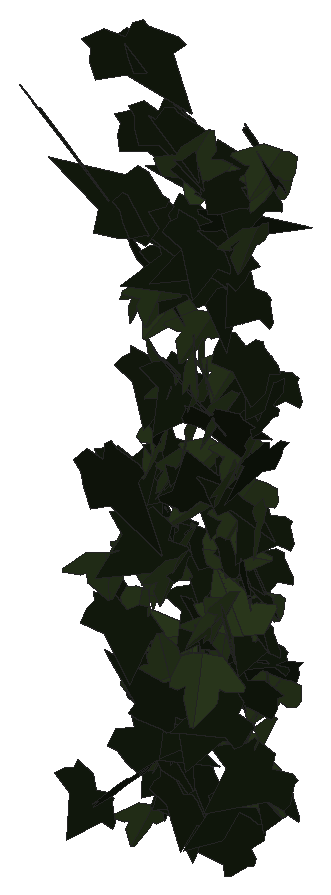
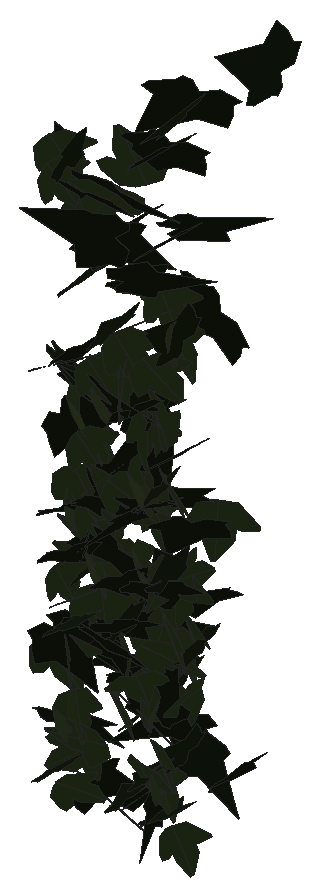
# SketchUp Ruby script. Lengths in inches.
U = 1.inch
M = Sketchup.active_model
def pt(a) = Geom::Point3d.new(a.map { |v| v * U })
def face(e, loops, mat)
  f = e.add_face(loops[0].map { |a| pt(a) })
  loops[1..].each { |l| e.add_face(l.map { |a| pt(a) }).erase! }
  f.material = f.back_material = mat if mat
  f
end
# faces: each face lists its corners as indices into pts; further lists are holes
def faces(e, pts, list, mat = nil) = list.each { |f| face(e, (f[0].is_a?(Array) ? f : [f]).map { |l| l.map { |i| pts[i] } }, mat) }
# xy, xz, yz: faces in a plane at the given z, y or x. An outline is a flat list of corners, or four numbers for a rectangle; further outlines are holes
def ring(l) = l.size == 4 ? [[l[0], l[1]], [l[2], l[1]], [l[2], l[3]], [l[0], l[3]]] : l.each_slice(2).to_a
def flat(e, list, mat, &to3) = list.each { |f| face(e, (f[0].is_a?(Array) ? f : [f]).map { |l| ring(l).map { |u, v| to3.(u, v) } }, mat) }
def xy(e, z, list, mat = nil) = flat(e, list, mat) { |x, y| [x, y, z] }
def xz(e, y, list, mat = nil) = flat(e, list, mat) { |x, z| [x, y, z] }
def yz(e, x, list, mat = nil) = flat(e, list, mat) { |y, z| [x, y, z] }
def lines(e, pts, list) = list.each { |a, b| e.add_line(pt(pts[a]), pt(pts[b])) }
# prism: a flat outline (further loops are holes) pulled along v
def prism(e, loops, v, mat = nil)
  f = face(e, loops, mat); d = Geom::Vector3d.new(v.map { |x| x * U })
  f.pushpull(f.normal.samedirection?(d) ? d.length : -d.length)
end
def box(e, o, s, mat = nil) = prism(e, [[o, [o[0] + s[0], o[1], o[2]], [o[0] + s[0], o[1] + s[1], o[2]], [o[0], o[1] + s[1], o[2]]]], [0, 0, s[2]], mat)
def at(x, y, z, deg = 0) = Geom::Transformation.translation(pt([x, y, z])) * Geom::Transformation.rotation(ORIGIN, Z_AXIS, deg.degrees)
def axes(o, x, y, z) = Geom::Transformation.new([*x, 0, *y, 0, *z, 0, *pt(o).to_a, 1])
def part(name) = M.definitions.add(name)
# library, detail: a bought-in or finely detailed component or shape, given as its bounding box
def library(name, o, s) = part(name).tap { |d| box(d.entities, o, s) }
def detail(e, o, s) = box(e.add_group.entities, o, s)
def put(e, d, t, mat = nil) = e.add_instance(d, t).tap { |i| i.material = mat if mat }
def group(e, t, mat = nil) = e.add_group.tap { |g| g.transformation = t; g.material = mat if mat }.entities
root = M.entities
M.materials.add("1026 AP 7946 SUNNY SIDE UP").color = [254, 231, 186]
M.materials.add("efeu1").color = [18, 25, 13]
M.materials.add("efeu2").color = [43, 57, 29]
c1 = part("ivyleaf_9")
p = [[1.54,2.16,1.25],[1.36,2.04,1.19],[-0.21,0.99,0.68],[-0.71,1.11,0.82],[-0.85,0.86,0.67],[-0.8,0.17,0.21],
  [-0.9,-0.01,0.1],[-0.67,-0.16,-0.02],[-0.08,-0.08,-0.05],[-0.03,-0.6,-0.4],[0.65,-0.88,-0.66],[0.83,-0.6,-0.49],
  [1.29,-0.42,-0.43],[1.8125,-0.07,-0.26],[1.21,0.44,0.15]]
faces(c1.entities,p,[[0,1,2,3,4,5,6,7,8,9,10,11,12,13,14]],"efeu1")
c2 = part("ivyleaf_10")
p = [[0,0.5,-0.03],[-0.0625,2.02,-0.43],[-0.19,2.01,-0.46],[-0.54,1.05,-0.29],[-0.52,0.625,-0.18],[-0.83,0.76,-0.28],
  [-1.16,0.64,-0.33],[-1.15,0.33,-0.24],[-0.77,-0.39,0.02],[-0.3,-0.51,0.16],[0.04,-0.48,0.23],[-0.02,2.01,-0.4375],
  [-0.06,2.01,-0.43],[0.04,-0.49,0.23],[0.67,-0.49,0.14],[1.38,0.36,-0.2],[1.375,0.51,-0.24],[0.81,0.65,-0.19],
  [0.62,0.59,-0.15],[0.6,1.09,-0.28],[0.5,1.23,-0.31]]
faces(c2.entities,p,[[0,1,2,3,4,5,6,7,8,9,10],[11,12,0,13,14,15,16,17,18,19,20]],"efeu2")
put(root,c1,axes([110.82,211.98,271.07],[0.22483,-0.24463,-0.03492],[-0.03089,0.02617,-0.29173],[0.3868,0.14428,-0.003]),"1026 AP 7946 SUNNY SIDE UP")
put(root,c1,axes([110.93,212.53,274.21],[-0.10088,-0.26489,0.10822],[-0.00053,-0.10914,-0.28036],[0.44895,-0.05965,0.02399]),"1026 AP 7946 SUNNY SIDE UP")
put(root,c1,axes([110.88,212.15,273.02],[-0.12749,-0.24464,-0.16443],[0.11207,0.14259,-0.26392],[0.44419,-0.10619,0.01939]),"1026 AP 7946 SUNNY SIDE UP")
put(root,c2,axes([111.05,212.09,272.0625],[0.02647,-0.03472,0.31078],[0.08986,-0.29657,-0.04015],[0.46926,0.05875,-0.00984]),"1026 AP 7946 SUNNY SIDE UP")
put(root,c1,axes([111.05,211.11,268.53],[-0.12847,-0.24075,0.1698],[-0.07523,-0.15923,-0.26279],[0.45379,-0.09456,0.00451]),"1026 AP 7946 SUNNY SIDE UP")
put(root,c1,axes([110.87,212.26,269.49],[0.16139,-0.23387,0.08171],[0.03475,-0.07829,-0.26334],[0.38743,0.10445,-0.01042]),"1026 AP 7946 SUNNY SIDE UP")
put(root,c2,axes([111.14,212.125,275.85],[0.01915,-0.31792,0.0495],[0.00358,-0.0498,-0.32805],[0.50599,0.01238,0.00045]),"1026 AP 7946 SUNNY SIDE UP")
put(root,c1,axes([111.45,211.65,277.25],[-0.30448,-0.25939,-0.13736],[-0.14977,-0.09316,0.33235],[-0.43234,0.21496,-0.01839]),"1026 AP 7946 SUNNY SIDE UP")
put(root,c2,axes([111.19,212.23,271.29],[0.24303,-0.2311,-0.07092],[-0.06134,0.05515,-0.28608],[0.37357,0.1594,-0.00084]),"1026 AP 7946 SUNNY SIDE UP")
put(root,c2,axes([111.08,211.8,270.11],[0.03825,-0.06161,-0.3049],[0.13909,0.28502,-0.05203],[0.45399,-0.08213,0.04163]),"1026 AP 7946 SUNNY SIDE UP")
put(root,c1,axes([110.875,212.39,276.02],[0.21679,-0.26213,0.13752],[0.08115,-0.12525,-0.30562],[0.45645,0.14677,-0.01098]),"1026 AP 7946 SUNNY SIDE UP")
put(root,c1,axes([110.97,212.55,272.3125],[0.02608,-0.19739,0.20165],[0.09253,-0.19029,-0.20278],[0.42847,0.05311,0.03151]),"1026 AP 7946 SUNNY SIDE UP")
put(root,c2,axes([111.25,212,267.9],[-0.15086,-0.24891,0.06861],[-0.02033,-0.06784,-0.27493],[0.40522,-0.09607,0.01175]),"1026 AP 7946 SUNNY SIDE UP")
put(root,c2,axes([111.3125,212.49,275.45],[-0.23769,-0.19774,0.18427],[-0.0587,-0.18912,-0.24746],[0.41633,-0.13956,0.07031]),"1026 AP 7946 SUNNY SIDE UP")
put(root,c1,axes([111.01,212.15,279.43],[0.23464,-0.27386,-0.07967],[-0.04055,0.07219,-0.32065],[0.44496,0.15099,0.0128]),"1026 AP 7946 SUNNY SIDE UP")
put(root,c1,axes([111.23,212.42,268.38],[-0.18187,-0.17107,0.16776],[0.00156,-0.18265,-0.19685],[0.37243,-0.08278,0.08275]),"1026 AP 7946 SUNNY SIDE UP")
put(root,c2,axes([111.39,211.96,271.86],[-0.50214,-0.04065,0.04773],[-0.06554,-0.03932,-0.33009],[0.07177,-0.32032,0.03253]),"1026 AP 7946 SUNNY SIDE UP")
put(root,c2,axes([111.33,212.25,268.89],[-0.00042,-0.29262,0.02638],[-0.00053,-0.02727,-0.30162],[0.46212,-0.0003,-0.00032]),"1026 AP 7946 SUNNY SIDE UP")
put(root,c1,axes([111.05,211.83,279.6],[-0.08354,-0.17438,-0.31942],[0.18521,0.28613,-0.18549],[0.52636,-0.12836,0.01457]),"1026 AP 7946 SUNNY SIDE UP")
put(root,c1,axes([111.27,212.48,272.05],[-0.2802,-0.22211,-0.04672],[0.06855,0.02141,-0.29248],[0.34941,-0.18232,0.01991]),"1026 AP 7946 SUNNY SIDE UP")
put(root,c2,axes([111.24,212.22,273.58],[0.32756,-0.2155,0.10995],[0.07975,-0.10029,-0.30768],[0.3705,0.21211,-0.03098]),"1026 AP 7946 SUNNY SIDE UP")
put(root,c2,axes([111.375,211.74,270.77],[0.10766,-0.28193,0.00565],[-0.00779,-0.0085,-0.29885],[0.44337,0.06831,-0.00662]),"1026 AP 7946 SUNNY SIDE UP")
put(root,c2,axes([111.4,212.24,269.3125],[0.2735,-0.1933,-0.0689],[-0.07163,0.0475,-0.26761],[0.31298,0.17979,-0.00103]),"1026 AP 7946 SUNNY SIDE UP")
put(root,c2,axes([111.35,212.06,272.08],[-0.10457,-0.21622,-0.22476],[0.10442,0.20654,-0.23183],[0.47016,-0.09396,0.0015]),"1026 AP 7946 SUNNY SIDE UP")
put(root,c2,axes([111.64,212.04,270.67],[-0.20058,0.01867,0.24939],[-0.29674,-0.17951,-0.08927],[0.23994,-0.20639,0.09807]),"1026 AP 7946 SUNNY SIDE UP")
put(root,c2,axes([111.27,211.74,271.24],[0.34499,-0.16401,0.14469],[0.14626,-0.11037,-0.28125],[0.30747,0.23652,-0.02856]),"1026 AP 7946 SUNNY SIDE UP")
put(root,c1,axes([111.59,211.15,268.87],[-0.16544,0.29418,-0.12402],[0.04198,-0.11994,-0.32224],[-0.49905,-0.10762,0.01401]),"1026 AP 7946 SUNNY SIDE UP")
put(root,c2,axes([111.1875,212.32,274.375],[-0.25193,0.10093,0.2724],[0.36559,-0.12516,0.19405],[0.25227,0.28217,-0.00918]),"1026 AP 7946 SUNNY SIDE UP")
put(root,c1,axes([111.02,210.1,279.2],[0.33578,-0.29164,0.19388],[0.1489,-0.16564,-0.37283],[0.52653,0.23283,-0.0182]),"1026 AP 7946 SUNNY SIDE UP")
put(root,c1,axes([111.53,212.12,268.46],[0.06782,-0.06736,-0.30721],[-0.34267,0.20388,-0.07883],[0.33629,0.22133,-0.01837]),"1026 AP 7946 SUNNY SIDE UP")
put(root,c1,axes([111.41,212.12,273.68],[0.03377,0.209,0.21516],[-0.14806,-0.19243,0.20841],[0.43898,-0.08098,0.05375]),"1026 AP 7946 SUNNY SIDE UP")
put(root,c2,axes([111.42,212.3,270.09],[-0.19323,0.22713,-0.09072],[0.04701,-0.08527,-0.26618],[-0.38089,-0.12575,0.01317]),"1026 AP 7946 SUNNY SIDE UP")
put(root,c1,axes([111.82,212.38,276.6],[-0.23655,0.01336,0.28194],[-0.41882,-0.08,-0.14732],[0.10055,-0.30181,0.04963]),"1026 AP 7946 SUNNY SIDE UP")
put(root,c1,axes([111.35,212.4375,273.39],[-0.0308,-0.22698,0.20443],[0.008,-0.20037,-0.23524],[0.47534,-0.01134,0.01721]),"1026 AP 7946 SUNNY SIDE UP")
put(root,c1,axes([111.29,211.77,270.31],[0.20454,-0.25715,-0.01721],[-0.02181,0.01006,-0.29671],[0.40446,0.13059,-0.0073]),"1026 AP 7946 SUNNY SIDE UP")
put(root,c2,axes([111.53,210.76,272.35],[-0.3134,-0.25493,-0.03631],[0.05081,0.01759,-0.33293],[0.40116,-0.20139,0.0138]),"1026 AP 7946 SUNNY SIDE UP")
put(root,c1,axes([111.54,212.125,269.84],[0.33563,-0.12698,0.14382],[-0.16714,0.09455,0.25527],[-0.24619,-0.2373,0.02275]),"1026 AP 7946 SUNNY SIDE UP")
put(root,c2,axes([111.55,212.26,274.41],[-0.16161,-0.27546,-0.04722],[0.0479,0.03582,-0.30224],[0.43607,-0.10602,0.01569]),"1026 AP 7946 SUNNY SIDE UP")
put(root,c2,axes([111.5,212.38,269.02],[0.38132,-0.11167,0.00637],[-0.00344,-0.02101,-0.27439],[0.17588,0.24169,-0.01919]),"1026 AP 7946 SUNNY SIDE UP")
put(root,c1,axes([111.45,211.29,271.29],[-0.14008,-0.29047,-0.03741],[0.04419,0.02757,-0.31224],[0.45784,-0.09153,0.01869]),"1026 AP 7946 SUNNY SIDE UP")
put(root,c1,axes([111.33,211.72,277.28],[0.19142,-0.2494,-0.13753],[0.00345,0.14468,-0.2785],[0.44375,0.10646,0.0615]),"1026 AP 7946 SUNNY SIDE UP")
put(root,c1,axes([111.38,212.36,269.02],[0.07782,-0.25434,0.06433],[0.0399,-0.06006,-0.26694],[0.41041,0.05406,0.01375]),"1026 AP 7946 SUNNY SIDE UP")
put(root,c1,axes([111.54,212.38,276.07],[-0.17902,-0.2306,0.14655],[-0.00973,-0.15343,-0.25983],[0.42702,-0.10017,0.05552]),"1026 AP 7946 SUNNY SIDE UP")
put(root,c1,axes([111.63,212.4,273.08],[-0.25672,-0.19054,0.14646],[-0.05548,-0.15239,-0.25115],[0.3707,-0.15476,0.06384]),"1026 AP 7946 SUNNY SIDE UP")
put(root,c2,axes([111.6875,211.74,276.12],[-0.18772,-0.27489,0.07302],[-0.01104,-0.0757,-0.30828],[0.44686,-0.11735,0.02306]),"1026 AP 7946 SUNNY SIDE UP")
put(root,c2,axes([111.66,212.12,273.32],[0.03751,-0.24578,0.1633],[0.0337,-0.15855,-0.25527],[0.45983,0.03167,0.00539]),"1026 AP 7946 SUNNY SIDE UP")
put(root,c2,axes([111.63,212.38,270.4],[0.28623,0.18692,-0.08485],[-0.05919,-0.07916,-0.26781],[-0.31636,0.18392,-0.02666]),"1026 AP 7946 SUNNY SIDE UP")
put(root,c2,axes([111.6,212.5,273.63],[0.14543,-0.19341,0.21253],[0.15147,-0.18376,-0.22186],[0.4194,0.13343,0.00643]),"1026 AP 7946 SUNNY SIDE UP")
put(root,c2,axes([111.64,212.14,269.93],[0.02505,-0.20313,0.22256],[0.12174,-0.20717,-0.20666],[0.45147,0.06713,0.04338]),"1026 AP 7946 SUNNY SIDE UP")
put(root,c2,axes([111.91,211.74,270.04],[-0.23993,-0.10944,0.2045],[-0.21514,-0.14725,-0.19224],[0.28526,-0.20311,0.02702]),"1026 AP 7946 SUNNY SIDE UP")
put(root,c1,axes([111.53,211.91,278.6],[0.12207,-0.29747,-0.09822],[0.02937,0.10077,-0.31321],[0.48949,0.06814,0.04329]),"1026 AP 7946 SUNNY SIDE UP")
put(root,c1,axes([111.51,211.46,269.48],[0.15298,-0.07527,-0.30834],[0.04638,0.31425,-0.0698],[0.48241,-0.00634,0.10449]),"1026 AP 7946 SUNNY SIDE UP")
put(root,c1,axes([111.75,212.22,268.43],[-0.16228,-0.1635,0.22591],[-0.08531,-0.21847,-0.19458],[0.42275,-0.10685,0.04746]),"1026 AP 7946 SUNNY SIDE UP")
put(root,c2,axes([111.77,212.18,272.17],[0.13474,-0.27024,0.06167],[0.02193,-0.05998,-0.29237],[0.43521,0.08669,-0.00436]),"1026 AP 7946 SUNNY SIDE UP")
put(root,c1,axes([111.62,212.125,269.88],[0.15844,-0.24429,-0.06255],[-0.03382,0.05531,-0.2719],[0.39383,0.10303,0.00182]),"1026 AP 7946 SUNNY SIDE UP")
put(root,c1,axes([111.83,212.21,274.51],[-0.26706,-0.24021,0.09302],[-0.06337,-0.08362,-0.30318],[0.39927,-0.17394,0.0141]),"1026 AP 7946 SUNNY SIDE UP")
put(root,c1,axes([111.59,211.76,278.57],[-0.15961,-0.16349,-0.25857],[0.23365,0.20149,-0.19667],[0.40755,-0.17954,0.01149]),"1026 AP 7946 SUNNY SIDE UP")
put(root,c1,axes([111.63,212.29,273.04],[0.18738,-0.21298,-0.21112],[-0.02491,0.2148,-0.23963],[0.46277,0.0978,0.07259]),"1026 AP 7946 SUNNY SIDE UP")
put(root,c2,axes([111.93,212.48,273.37],[-0.11937,-0.18452,0.20834],[-0.00682,-0.21008,-0.19935],[0.43163,-0.05435,0.05447]),"1026 AP 7946 SUNNY SIDE UP")
put(root,c1,axes([112.1,212.04,276.4],[-0.32009,-0.11493,0.21395],[-0.26172,-0.12713,-0.24055],[0.26734,-0.26207,0.02067]),"1026 AP 7946 SUNNY SIDE UP")
put(root,c1,axes([111.73,212.5,268.5625],[-0.00014,-0.22901,0.13946],[0.03343,-0.13624,-0.23597],[0.41801,0.01082,0.01892]),"1026 AP 7946 SUNNY SIDE UP")
put(root,c1,axes([112.1,211.83,269.51],[-0.37902,0.09805,-0.12857],[-0.16891,0.06764,0.26769],[0.18465,0.26314,-0.01904]),"1026 AP 7946 SUNNY SIDE UP")
put(root,c2,axes([111.96,211.56,270.49],[-0.26277,-0.24162,-0.09915],[-0.11075,-0.0664,0.30161],[-0.39285,0.18033,-0.01871]),"1026 AP 7946 SUNNY SIDE UP")
put(root,c2,axes([112.01,212.26,275.48],[-0.16254,-0.28346,0.12639],[-0.04011,-0.12279,-0.31107],[0.48502,-0.10515,0.01663]),"1026 AP 7946 SUNNY SIDE UP")
put(root,c1,axes([111.87,212.46,271.97],[-0.15591,-0.2612,-0.0103],[0.00561,0.00775,-0.28778],[0.41089,-0.09922,0.00002]),"1026 AP 7946 SUNNY SIDE UP")
put(root,c1,axes([112.11,211.27,272.62],[-0.37106,-0.17084,0.15162],[-0.15554,-0.11456,-0.29909],[0.31973,-0.25399,0.03046]),"1026 AP 7946 SUNNY SIDE UP")
put(root,c1,axes([111.63,212.13,274.54],[0.18476,-0.21631,0.23673],[0.18997,-0.19711,-0.25459],[0.45995,0.1683,0.01006]),"1026 AP 7946 SUNNY SIDE UP")
put(root,c1,axes([112.06,212.39,271.13],[-0.30877,-0.18908,0.04464],[-0.01532,-0.05348,-0.27928],[0.30501,-0.1941,0.03117]),"1026 AP 7946 SUNNY SIDE UP")
put(root,c2,axes([112.14,212.18,272.94],[-0.08976,-0.17585,0.25529],[-0.08015,-0.24405,-0.19118],[0.47232,-0.07483,0.01608]),"1026 AP 7946 SUNNY SIDE UP")
put(root,c2,axes([111.91,212.29,270.63],[-0.1431,0.14098,-0.22482],[0.09113,-0.21524,-0.16879],[-0.39932,-0.09964,0.04205]),"1026 AP 7946 SUNNY SIDE UP")
put(root,c1,axes([111.92,211.99,268.36],[-0.05851,-0.27502,-0.01601],[0.00027,0.01409,-0.28581],[0.433,-0.03717,-0.00198]),"1026 AP 7946 SUNNY SIDE UP")
put(root,c2,axes([112.07,212.29,269.88],[0.25731,-0.21599,-0.00995],[-0.02768,-0.00278,-0.27871],[0.33876,0.16383,-0.01522]),"1026 AP 7946 SUNNY SIDE UP")
put(root,c1,axes([111.93,211.87,268.42],[-0.03632,-0.2562,0.13242],[0.0097,-0.13083,-0.26526],[0.45163,-0.01779,0.01634]),"1026 AP 7946 SUNNY SIDE UP")
put(root,c1,axes([112.07,212.49,273.11],[-0.27728,-0.22148,-0.07883],[0.10417,0.0431,-0.29034],[0.35275,-0.18682,0.02378]),"1026 AP 7946 SUNNY SIDE UP")
put(root,c1,axes([112.4375,211.02,270.22],[0.03702,0.01065,0.32016],[-0.41959,0.16058,0.0161],[-0.25084,-0.26704,0.02032]),"1026 AP 7946 SUNNY SIDE UP")
put(root,c2,axes([112.26,211.92,275],[-0.23218,0.19916,0.20585],[-0.20283,0.15149,-0.2543],[-0.39311,-0.19579,0.00963]),"1026 AP 7946 SUNNY SIDE UP")
put(root,c2,axes([112.07,211.82,278],[-0.27727,-0.26926,0.07668],[0.04714,0.07109,0.33171],[-0.43738,0.17836,-0.01286]),"1026 AP 7946 SUNNY SIDE UP")
put(root,c1,axes([111.98,212.51,275.83],[0.03637,-0.27324,0.12538],[0.02924,-0.12208,-0.2831],[0.47042,0.02872,0.0079]),"1026 AP 7946 SUNNY SIDE UP")
put(root,c2,axes([112.2,211.97,274.79],[0.04473,-0.24829,-0.1799],[0.00766,0.17434,-0.2556],[0.47598,0.02052,0.02102]),"1026 AP 7946 SUNNY SIDE UP")
put(root,c1,axes([112.17,211.95,272.98],[0.29177,0.13608,0.24442],[-0.33379,-0.10767,0.23478],[0.26952,-0.28065,0.02617]),"1026 AP 7946 SUNNY SIDE UP")
put(root,c1,axes([112.59,212.2,277.76],[-0.33781,0.11245,0.21123],[-0.32853,0.03086,-0.24355],[-0.16318,-0.29492,0.05305]),"1026 AP 7946 SUNNY SIDE UP")
put(root,c1,axes([112.18,212.42,270.85],[-0.35646,-0.08487,-0.13997],[0.23423,-0.02721,-0.23955],[0.09093,-0.26264,0.06833]),"1026 AP 7946 SUNNY SIDE UP")
put(root,c1,axes([112.1,212.18,270.94],[-0.07725,-0.13619,0.25428],[0.03268,-0.25237,-0.14023],[0.44312,-0.00513,0.05467]),"1026 AP 7946 SUNNY SIDE UP")
put(root,c2,axes([112.35,211.15,272.39],[-0.03818,-0.32615,0.01372],[0.00385,-0.01539,-0.33699],[0.51337,-0.02414,0.00355]),"1026 AP 7946 SUNNY SIDE UP")
put(root,c1,axes([112.36,211.66,269.95],[-0.26941,-0.20251,0.0725],[-0.05169,-0.06569,-0.27312],[0.33372,-0.17366,0.01622]),"1026 AP 7946 SUNNY SIDE UP")
put(root,c1,axes([112.73,212.16,274.49],[-0.24201,0.12767,0.24973],[-0.33222,0.1204,-0.20343],[-0.27267,-0.26001,0.02621]),"1026 AP 7946 SUNNY SIDE UP")
put(root,c1,axes([112.55,211.99,276.87],[0.00963,-0.00479,-0.32525],[-0.08306,-0.31132,0.00199],[-0.48945,0.05274,-0.00674]),"1026 AP 7946 SUNNY SIDE UP")
put(root,c2,axes([112.45,212.32,274.98],[-0.17984,-0.24315,0.1331],[-0.01654,-0.13741,-0.27388],[0.43366,-0.10608,0.04475]),"1026 AP 7946 SUNNY SIDE UP")
put(root,c1,axes([112.08,212.31,272.27],[-0.01393,-0.11467,-0.27757],[0.42599,0.09758,-0.05151],[0.17224,-0.2506,0.10496]),"1026 AP 7946 SUNNY SIDE UP")
put(root,c1,axes([112.32,211.81,277.05],[-0.08481,-0.28227,0.11358],[-0.01217,-0.11229,-0.29643],[0.47726,-0.05302,0.01262]),"1026 AP 7946 SUNNY SIDE UP")
put(root,c2,axes([112.18,212.18,277.76],[0.35832,0.16931,0.15914],[0.21441,0.07325,-0.29133],[-0.28839,0.26482,-0.01887]),"1026 AP 7946 SUNNY SIDE UP")
put(root,c2,axes([112.52,212.36,272.75],[-0.0822,-0.25244,0.1452],[0.0235,-0.14683,-0.2634],[0.45511,-0.03801,0.03982]),"1026 AP 7946 SUNNY SIDE UP")
put(root,c2,axes([112.59,211.99,271.2],[-0.35775,-0.21522,0.02764],[-0.0036,-0.03826,-0.32174],[0.34126,-0.22602,0.02558]),"1026 AP 7946 SUNNY SIDE UP")
put(root,c1,axes([112.31,212.16,270.73],[-0.13481,-0.0292,-0.27614],[0.42219,0.01457,-0.09008],[0.03591,-0.28089,0.02237]),"1026 AP 7946 SUNNY SIDE UP")
put(root,c1,axes([112.33,212.16,273.29],[0.24945,-0.23281,-0.15072],[-0.05179,0.1501,-0.28457],[0.42813,0.15381,0.05339]),"1026 AP 7946 SUNNY SIDE UP")
put(root,c2,axes([112.57,212.05,274.53],[0.09134,-0.2676,0.19315],[0.03684,-0.18807,-0.28283],[0.51382,0.06105,-0.01406]),"1026 AP 7946 SUNNY SIDE UP")
put(root,c2,axes([112.72,212.34,273.19],[-0.34615,-0.16137,0.11785],[-0.11724,-0.09231,-0.28025],[0.28899,-0.23074,0.02747]),"1026 AP 7946 SUNNY SIDE UP")
put(root,c2,axes([112.64,212.32,273.76],[-0.14002,-0.24517,0.14775],[0.01033,-0.15345,-0.26439],[0.44761,-0.07315,0.05232]),"1026 AP 7946 SUNNY SIDE UP")
put(root,c1,axes([112.59,211.58,270.04],[-0.28851,-0.20425,-0.02535],[0.05347,0.00084,-0.2817],[0.31882,-0.18497,0.02431]),"1026 AP 7946 SUNNY SIDE UP")
put(root,c1,axes([112.24,212.22,277.09],[0.24178,0.16705,-0.22412],[0.19767,0.17996,0.23394],[0.38466,-0.19748,0.02065]),"1026 AP 7946 SUNNY SIDE UP")
put(root,c1,axes([112.66,212.17,268.35],[0.00609,-0.04922,-0.31304],[0.13249,-0.29182,0.04814],[-0.46509,-0.08378,0.00962]),"1026 AP 7946 SUNNY SIDE UP")
put(root,c2,axes([112.66,212.14,271.9],[0.13779,-0.28604,0.02327],[-0.00175,-0.02566,-0.30822],[0.45137,0.08722,-0.0083]),"1026 AP 7946 SUNNY SIDE UP")
put(root,c2,axes([112.75,212.54,268.39],[-0.1702,-0.08994,0.24023],[-0.07428,-0.24269,-0.12018],[0.38667,-0.08621,0.08265]),"1026 AP 7946 SUNNY SIDE UP")
put(root,c2,axes([112.3,212.18,272.15],[0.11213,-0.07735,-0.28598],[0.42772,-0.07501,0.09323],[-0.14757,-0.27618,0.05292]),"1026 AP 7946 SUNNY SIDE UP")
put(root,c1,axes([112.56,211.74,274.45],[0.45869,0.11294,-0.06624],[-0.08013,-0.04765,-0.32147],[-0.18853,0.29503,-0.02453]),"1026 AP 7946 SUNNY SIDE UP")
put(root,c1,axes([112.61,212.37,277.73],[-0.35136,-0.16292,-0.12492],[0.24084,-0.01867,-0.26706],[0.2084,-0.25311,0.09801]),"1026 AP 7946 SUNNY SIDE UP")
put(root,c2,axes([112.72,212.33,269.67],[-0.01851,-0.27072,-0.05966],[-0.00083,0.05644,-0.27881],[0.43481,-0.01142,-0.00307]),"1026 AP 7946 SUNNY SIDE UP")
put(root,c2,axes([112.73,211.85,273.58],[0.10816,-0.28905,0.00472],[-0.00966,-0.00786,-0.30603],[0.4545,0.06862,-0.00763]),"1026 AP 7946 SUNNY SIDE UP")
put(root,c1,axes([112.54,212.28,272.24],[0.19031,-0.27685,-0.09087],[-0.04073,0.08319,-0.31065],[0.45432,0.12343,0.01021]),"1026 AP 7946 SUNNY SIDE UP")
put(root,c2,axes([112.4375,212.375,269.13],[-0.11572,-0.02412,-0.27143],[0.39841,-0.08467,-0.06545],[-0.11901,-0.25999,0.0448]),"1026 AP 7946 SUNNY SIDE UP")
put(root,c1,axes([112.6,212.16,271.78],[0.1728,-0.27106,-0.02524],[-0.02353,0.01871,-0.30113],[0.42709,0.1107,-0.00638]),"1026 AP 7946 SUNNY SIDE UP")
put(root,c1,axes([112.67,212.3,275.27],[-0.01052,-0.30286,-0.02139],[-0.00774,0.01915,-0.31192],[0.4771,-0.00637,-0.00553]),"1026 AP 7946 SUNNY SIDE UP")
put(root,c1,axes([112.75,212.51,272.11],[-0.18197,-0.26582,0.01692],[0.00457,-0.02081,-0.29858],[0.41891,-0.11524,0.0106]),"1026 AP 7946 SUNNY SIDE UP")
put(root,c1,axes([113.13,211.76,268.11],[-0.3194,0.18957,0.10487],[-0.14635,0.04718,-0.28458],[-0.30417,-0.22177,0.0268]),"1026 AP 7946 SUNNY SIDE UP")
put(root,c1,axes([112.76,212.31,276.22],[-0.1403,-0.20986,0.22193],[-0.04324,-0.2193,-0.23183],[0.47227,-0.08242,0.04471]),"1026 AP 7946 SUNNY SIDE UP")
put(root,c2,axes([112.79,211.55,271.6],[0.04491,-0.08881,0.30836],[0.08635,-0.29497,-0.09712],[0.48405,0.06086,-0.01128]),"1026 AP 7946 SUNNY SIDE UP")
put(root,c1,axes([113.05,211.81,270.59],[0.14562,0.06956,-0.27787],[-0.2729,-0.20845,-0.11782],[-0.34336,0.19517,-0.0242]),"1026 AP 7946 SUNNY SIDE UP")
put(root,c2,axes([112.88,211.71,271.79],[0.03782,-0.27194,0.11809],[0.03218,-0.11474,-0.28175],[0.46387,0.03014,0.00992]),"1026 AP 7946 SUNNY SIDE UP")
put(root,c1,axes([112.47,209.57,274.66],[-0.09183,-0.06074,-0.40889],[0.62253,0.05603,-0.06858],[0.10193,-0.3969,0.05047]),"1026 AP 7946 SUNNY SIDE UP")
put(root,c1,axes([112.88,212.49,272.73],[-0.24753,-0.21669,0.09124],[-0.00957,-0.10433,-0.27098],[0.3687,-0.14818,0.05422]),"1026 AP 7946 SUNNY SIDE UP")
put(root,c2,axes([112.95,212.07,277.21],[-0.08757,-0.30268,0.03345],[-0.00118,-0.03462,-0.31721],[0.47896,-0.05542,0.00533]),"1026 AP 7946 SUNNY SIDE UP")
put(root,c1,axes([112.88,212.5,270.83],[-0.20377,-0.168,0.18222],[-0.0101,-0.19884,-0.1995],[0.38454,-0.09424,0.09132]),"1026 AP 7946 SUNNY SIDE UP")
put(root,c1,axes([112.8,212.14,271.97],[-0.02783,-0.0023,0.34086],[-0.05279,-0.32963,-0.00614],[0.51761,-0.03374,0.0177]),"1026 AP 7946 SUNNY SIDE UP")
put(root,c1,axes([112.85,212.21,271.2],[-0.14817,-0.24301,0.09758],[0.02017,-0.10633,-0.26468],[0.41041,-0.08251,0.04824]),"1026 AP 7946 SUNNY SIDE UP")
put(root,c2,axes([112.88,212.52,269.51],[0.08511,-0.20022,0.19811],[0.09856,-0.18324,-0.21453],[0.42653,0.08229,0.01004]),"1026 AP 7946 SUNNY SIDE UP")
put(root,c2,axes([112.75,212.24,268.84],[-0.33479,-0.00288,-0.17099],[0.25912,-0.03592,-0.21737],[-0.03119,-0.26755,0.02943]),"1026 AP 7946 SUNNY SIDE UP")
put(root,c2,axes([112.875,211.57,271.6875],[-0.20183,0.28018,-0.06184],[0.02157,-0.06143,-0.31757],[-0.45056,-0.12845,0.0125]),"1026 AP 7946 SUNNY SIDE UP")
put(root,c2,axes([112.9,211.08,271.04],[0.24737,0.31698,-0.1089],[-0.06843,-0.09841,-0.3651],[-0.52184,0.16316,-0.00374]),"1026 AP 7946 SUNNY SIDE UP")
put(root,c1,axes([113.09,212.28,270.59],[-0.00016,0.2124,-0.20796],[-0.0049,-0.20306,-0.21999],[-0.46203,0.00208,0.00241]),"1026 AP 7946 SUNNY SIDE UP")
put(root,c2,axes([113.03,211.67,271.55],[0.36883,0.20328,0.06689],[-0.10716,-0.01828,0.31814],[0.31739,-0.2424,0.02968]),"1026 AP 7946 SUNNY SIDE UP")
put(root,c2,axes([112.95,212.125,274.16],[0.1783,-0.2316,0.15464],[0.07588,-0.14458,-0.26589],[0.42842,0.12199,-0.01726]),"1026 AP 7946 SUNNY SIDE UP")
put(root,c2,axes([112.84,212.4,272.76],[0.08641,-0.14015,0.25884],[0.22298,-0.21029,-0.15354],[0.39486,0.14942,0.03006]),"1026 AP 7946 SUNNY SIDE UP")
put(root,c2,axes([113.03,212.46,277.91],[-0.12351,-0.24996,0.16759],[0.02619,-0.17306,-0.26437],[0.46944,-0.05611,0.05884]),"1026 AP 7946 SUNNY SIDE UP")
put(root,c2,axes([113.14,212.31,270.33],[-0.32378,-0.20106,0.12807],[-0.09599,-0.11558,-0.29474],[0.36006,-0.21162,0.03658]),"1026 AP 7946 SUNNY SIDE UP")
put(root,c1,axes([112.8,212.51,278.17],[0.01165,-0.17129,0.26152],[0.08244,-0.25046,-0.17647],[0.47572,0.0476,0.02418]),"1026 AP 7946 SUNNY SIDE UP")
put(root,c2,axes([113.1,212.35,278.29],[-0.24064,-0.2226,0.14233],[-0.02601,-0.15288,-0.27105],[0.41219,-0.13961,0.06599]),"1026 AP 7946 SUNNY SIDE UP")
put(root,c1,axes([112.99,212.5,274.95],[-0.2343,-0.22483,0.11161],[0.01124,-0.13137,-0.26834],[0.39314,-0.13023,0.07419]),"1026 AP 7946 SUNNY SIDE UP")
put(root,c2,axes([113.08,212.16,270.36],[0.1415,-0.2358,-0.16129],[-0.0546,0.15243,-0.25841],[0.44053,0.09463,0.01978]),"1026 AP 7946 SUNNY SIDE UP")
put(root,c1,axes([112.94,212.58,268.6],[-0.10465,-0.22348,0.15985],[0.01544,-0.16288,-0.23637],[0.42866,-0.04869,0.04754]),"1026 AP 7946 SUNNY SIDE UP")
put(root,c1,axes([113.29,212.03,274.76],[-0.36619,0.21153,-0.04338],[0.02521,-0.04659,-0.32348],[-0.33858,-0.23225,0.02284]),"1026 AP 7946 SUNNY SIDE UP")
put(root,c2,axes([113.05,212.32,271.54],[-0.1037,-0.23409,0.13494],[0.06114,-0.14311,-0.2417],[0.41838,-0.03711,0.06877]),"1026 AP 7946 SUNNY SIDE UP")
put(root,c1,axes([113.23,212.08,269.18],[-0.47105,-0.10157,0.04052],[-0.0421,-0.04464,-0.32432],[0.16635,-0.29891,0.03267]),"1026 AP 7946 SUNNY SIDE UP")
put(root,c2,axes([112.79,210.99,275.76],[0.07786,-0.02173,0.35221],[0.37504,-0.24594,-0.05311],[0.38692,0.24276,-0.01939]),"1026 AP 7946 SUNNY SIDE UP")
put(root,c1,axes([113.21,211.39,270.33],[-0.26183,-0.12057,0.19479],[-0.20639,-0.1396,-0.21084],[0.28703,-0.21036,0.02609]),"1026 AP 7946 SUNNY SIDE UP")
put(root,c1,axes([113.13,212.17,273.94],[-0.13115,0.15611,-0.25141],[0.15775,-0.22366,-0.18337],[-0.4286,-0.13009,0.00944]),"1026 AP 7946 SUNNY SIDE UP")
